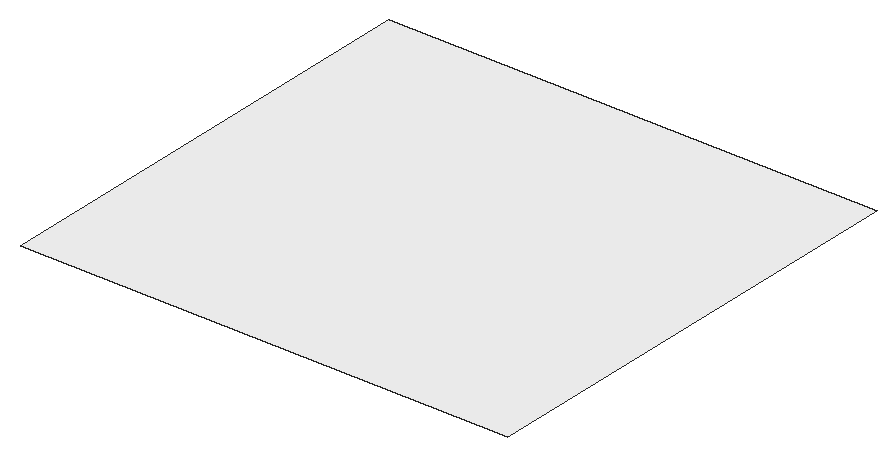
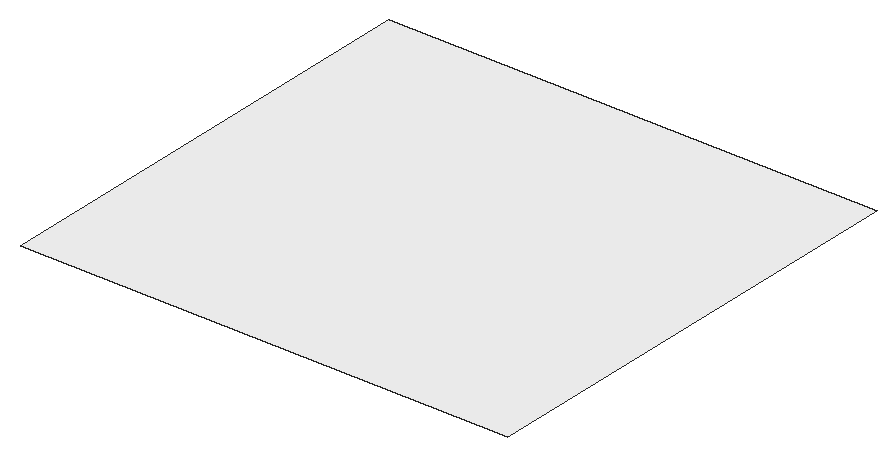
# SketchUp Ruby script. Lengths in inches.
U = 1.inch
M = Sketchup.active_model
def pt(a) = Geom::Point3d.new(a.map { |v| v * U })
def face(e, loops, mat)
  f = e.add_face(loops[0].map { |a| pt(a) })
  loops[1..].each { |l| e.add_face(l.map { |a| pt(a) }).erase! }
  f.material = f.back_material = mat if mat
  f
end
# faces: each face lists its corners as indices into pts; further lists are holes
def faces(e, pts, list, mat = nil) = list.each { |f| face(e, (f[0].is_a?(Array) ? f : [f]).map { |l| l.map { |i| pts[i] } }, mat) }
# xy, xz, yz: faces in a plane at the given z, y or x. An outline is a flat list of corners, or four numbers for a rectangle; further outlines are holes
def ring(l) = l.size == 4 ? [[l[0], l[1]], [l[2], l[1]], [l[2], l[3]], [l[0], l[3]]] : l.each_slice(2).to_a
def flat(e, list, mat, &to3) = list.each { |f| face(e, (f[0].is_a?(Array) ? f : [f]).map { |l| ring(l).map { |u, v| to3.(u, v) } }, mat) }
def xy(e, z, list, mat = nil) = flat(e, list, mat) { |x, y| [x, y, z] }
def xz(e, y, list, mat = nil) = flat(e, list, mat) { |x, z| [x, y, z] }
def yz(e, x, list, mat = nil) = flat(e, list, mat) { |y, z| [x, y, z] }
def lines(e, pts, list) = list.each { |a, b| e.add_line(pt(pts[a]), pt(pts[b])) }
# prism: a flat outline (further loops are holes) pulled along v
def prism(e, loops, v, mat = nil)
  f = face(e, loops, mat); d = Geom::Vector3d.new(v.map { |x| x * U })
  f.pushpull(f.normal.samedirection?(d) ? d.length : -d.length)
end
def box(e, o, s, mat = nil) = prism(e, [[o, [o[0] + s[0], o[1], o[2]], [o[0] + s[0], o[1] + s[1], o[2]], [o[0], o[1] + s[1], o[2]]]], [0, 0, s[2]], mat)
def at(x, y, z, deg = 0) = Geom::Transformation.translation(pt([x, y, z])) * Geom::Transformation.rotation(ORIGIN, Z_AXIS, deg.degrees)
def axes(o, x, y, z) = Geom::Transformation.new([*x, 0, *y, 0, *z, 0, *pt(o).to_a, 1])
def part(name) = M.definitions.add(name)
# library, detail: a bought-in or finely detailed component or shape, given as its bounding box
def library(name, o, s) = part(name).tap { |d| box(d.entities, o, s) }
def detail(e, o, s) = box(e.add_group.entities, o, s)
def put(e, d, t, mat = nil) = e.add_instance(d, t).tap { |i| i.material = mat if mat }
def group(e, t, mat = nil) = e.add_group.tap { |g| g.transformation = t; g.material = mat if mat }.entities
root = M.entities
M.materials.add("Dado").color = [252, 229, 201]
M.materials.add("[Color M00]").color = [255, 255, 255]
xy(root,120,[[29,128,114,133]],"[Color M00]")
xy(root,121,[[29,20,114,20,114,133,112.5,133,112.5,21.5,30.5,21.5,30.5,133,29,133]],"[Color M00]")
xy(root,122,[[14.87,17,14.68,17.02,14.5,17.04,14.3125,17.08,14.13,17.13,13.95,17.1875,13.78,17.26,13.61,17.34,13.44,17.43,13.14,17.65,12.99,17.77,12.86,17.9,12.73,18.04,12.61,18.1875,12.5,18.34,12.4,18.5,12.3125,18.67,12.23,18.84,12.17,19.02,12.11,19.19,12.07,19.38,12.03,19.5625,12.01,19.75,12,19.9375,12,20.13,12.02,20.32,12.04,20.5,12.08,20.6875,12.13,20.87,12.1875,21.05,12.26,21.22,12.34,21.39,12.43,21.56,12.65,21.86,12.77,22.01,12.9,22.14,13.04,22.27,13.1875,22.39,13.34,22.5,13.5,22.6,13.67,22.6875,13.84,22.77,14.02,22.83,14.19,22.89,14.38,22.93,14.5625,22.97,14.75,22.99,14.9375,23,15.13,23,15.32,22.98,15.5,22.96,15.6875,22.92,15.87,22.87,16.05,22.8125,16.22,22.74,16.39,22.66,16.56,22.57,16.86,22.35,17.01,22.23,17.14,22.1,17.27,21.96,17.39,21.8125,17.5,21.66,17.6,21.5,17.6875,21.33,17.77,21.16,17.83,20.98,17.89,20.81,17.93,20.62,17.97,20.4375,17.99,20.25,18,20.0625,18,19.87,17.98,19.68,17.96,19.5,17.92,19.3125,17.87,19.13,17.8125,18.95,17.74,18.78,17.66,18.61,17.57,18.44,17.35,18.14,17.23,17.99,17.1,17.86,16.96,17.73,16.8125,17.61,16.66,17.5,16.5,17.4,16.33,17.3125,16.16,17.23,15.98,17.17,15.81,17.11,15.62,17.07,15.4375,17.03,15.25,17.01,15.0625,17],[127.87,17,127.68,17.02,127.5,17.04,127.3125,17.08,127.13,17.13,126.95,17.1875,126.78,17.26,126.61,17.34,126.44,17.43,126.14,17.65,125.99,17.77,125.86,17.9,125.73,18.04,125.61,18.1875,125.5,18.34,125.4,18.5,125.3125,18.67,125.23,18.84,125.17,19.02,125.11,19.19,125.07,19.38,125.03,19.5625,125.01,19.75,125,19.9375,125,20.13,125.02,20.32,125.04,20.5,125.08,20.6875,125.13,20.87,125.1875,21.05,125.26,21.22,125.34,21.39,125.43,21.56,125.65,21.86,125.77,22.01,125.9,22.14,126.04,22.27,126.1875,22.39,126.34,22.5,126.5,22.6,126.67,22.6875,126.84,22.77,127.02,22.83,127.19,22.89,127.38,22.93,127.5625,22.97,127.75,22.99,127.9375,23,128.13,23,128.32,22.98,128.5,22.96,128.6875,22.92,128.87,22.87,129.05,22.8125,129.22,22.74,129.39,22.66,129.56,22.57,129.86,22.35,130.01,22.23,130.14,22.1,130.27,21.96,130.39,21.8125,130.5,21.66,130.6,21.5,130.6875,21.33,130.77,21.16,130.83,20.98,130.89,20.81,130.93,20.62,130.97,20.4375,130.99,20.25,131,20.0625,131,19.87,130.98,19.68,130.96,19.5,130.92,19.3125,130.87,19.13,130.8125,18.95,130.74,18.78,130.66,18.61,130.57,18.44,130.35,18.14,130.23,17.99,130.1,17.86,129.96,17.73,129.8125,17.61,129.66,17.5,129.5,17.4,129.33,17.3125,129.16,17.23,128.98,17.17,128.81,17.11,128.62,17.07,128.4375,17.03,128.25,17.01,128.0625,17],[14.87,61,14.68,61.02,14.5,61.04,14.3125,61.08,14.13,61.13,13.95,61.1875,13.78,61.26,13.61,61.34,13.44,61.43,13.14,61.65,12.99,61.77,12.86,61.9,12.73,62.04,12.61,62.1875,12.5,62.34,12.4,62.5,12.3125,62.67,12.23,62.84,12.17,63.02,12.11,63.19,12.07,63.38,12.03,63.5625,12.01,63.75,12,63.9375,12,64.13,12.02,64.32,12.04,64.5,12.08,64.6875,12.13,64.87,12.1875,65.05,12.26,65.22,12.34,65.39,12.43,65.56,12.65,65.86,12.77,66.01,12.9,66.14,13.04,66.27,13.1875,66.39,13.34,66.5,13.5,66.6,13.67,66.6875,13.84,66.77,14.02,66.83,14.19,66.89,14.38,66.93,14.5625,66.97,14.75,66.99,14.9375,67,15.13,67,15.32,66.98,15.5,66.96,15.6875,66.92,15.87,66.87,16.05,66.8125,16.22,66.74,16.39,66.66,16.56,66.57,16.86,66.35,17.01,66.23,17.14,66.1,17.27,65.96,17.39,65.8125,17.5,65.66,17.6,65.5,17.6875,65.33,17.77,65.16,17.83,64.98,17.89,64.81,17.93,64.62,17.97,64.4375,17.99,64.25,18,64.0625,18,63.87,17.98,63.68,17.96,63.5,17.92,63.3125,17.87,63.13,17.8125,62.95,17.74,62.78,17.66,62.61,17.57,62.44,17.35,62.14,17.23,61.99,17.1,61.86,16.96,61.73,16.8125,61.61,16.66,61.5,16.5,61.4,16.33,61.3125,16.16,61.23,15.98,61.17,15.81,61.11,15.62,61.07,15.4375,61.03,15.25,61.01,15.0625,61],[127.87,61,127.68,61.02,127.5,61.04,127.3125,61.08,127.13,61.13,126.95,61.1875,126.78,61.26,126.61,61.34,126.44,61.43,126.14,61.65,125.99,61.77,125.86,61.9,125.73,62.04,125.61,62.1875,125.5,62.34,125.4,62.5,125.3125,62.67,125.23,62.84,125.17,63.02,125.11,63.19,125.07,63.38,125.03,63.5625,125.01,63.75,125,63.9375,125,64.13,125.02,64.32,125.04,64.5,125.08,64.6875,125.13,64.87,125.1875,65.05,125.26,65.22,125.34,65.39,125.43,65.56,125.65,65.86,125.77,66.01,125.9,66.14,126.04,66.27,126.1875,66.39,126.34,66.5,126.5,66.6,126.67,66.6875,126.84,66.77,127.02,66.83,127.19,66.89,127.38,66.93,127.5625,66.97,127.75,66.99,127.9375,67,128.13,67,128.32,66.98,128.5,66.96,128.6875,66.92,128.87,66.87,129.05,66.8125,129.22,66.74,129.39,66.66,129.56,66.57,129.86,66.35,130.01,66.23,130.14,66.1,130.27,65.96,130.39,65.8125,130.5,65.66,130.6,65.5,130.6875,65.33,130.77,65.16,130.83,64.98,130.89,64.81,130.93,64.62,130.97,64.4375,130.99,64.25,131,64.0625,131,63.87,130.98,63.68,130.96,63.5,130.92,63.3125,130.87,63.13,130.8125,62.95,130.74,62.78,130.66,62.61,130.57,62.44,130.35,62.14,130.23,61.99,130.1,61.86,129.96,61.73,129.8125,61.61,129.66,61.5,129.5,61.4,129.33,61.3125,129.16,61.23,128.98,61.17,128.81,61.11,128.62,61.07,128.4375,61.03,128.25,61.01,128.0625,61],[14.87,105,14.68,105.02,14.5,105.04,14.3125,105.08,14.13,105.13,13.95,105.1875,13.78,105.26,13.61,105.34,13.44,105.43,13.14,105.65,12.99,105.77,12.86,105.9,12.73,106.04,12.61,106.1875,12.5,106.34,12.4,106.5,12.3125,106.67,12.23,106.84,12.17,107.02,12.11,107.19,12.07,107.38,12.03,107.5625,12.01,107.75,12,107.9375,12,108.13,12.02,108.32,12.04,108.5,12.08,108.6875,12.13,108.87,12.1875,109.05,12.26,109.22,12.34,109.39,12.43,109.56,12.65,109.86,12.77,110.01,12.9,110.14,13.04,110.27,13.1875,110.39,13.34,110.5,13.5,110.6,13.67,110.6875,13.84,110.77,14.02,110.83,14.19,110.89,14.38,110.93,14.5625,110.97,14.75,110.99,14.9375,111,15.13,111,15.32,110.98,15.5,110.96,15.6875,110.92,15.87,110.87,16.05,110.8125,16.22,110.74,16.39,110.66,16.56,110.57,16.86,110.35,17.01,110.23,17.14,110.1,17.27,109.96,17.39,109.8125,17.5,109.66,17.6,109.5,17.6875,109.33,17.77,109.16,17.83,108.98,17.89,108.81,17.93,108.62,17.97,108.4375,17.99,108.25,18,108.0625,18,107.87,17.98,107.68,17.96,107.5,17.92,107.3125,17.87,107.13,17.8125,106.95,17.74,106.78,17.66,106.61,17.57,106.44,17.35,106.14,17.23,105.99,17.1,105.86,16.96,105.73,16.8125,105.61,16.66,105.5,16.5,105.4,16.33,105.3125,16.16,105.23,15.98,105.17,15.81,105.11,15.62,105.07,15.4375,105.03,15.25,105.01,15.0625,105],
  [127.87,105,127.68,105.02,127.5,105.04,127.3125,105.08,127.13,105.13,126.95,105.1875,126.78,105.26,126.61,105.34,126.44,105.43,126.14,105.65,125.99,105.77,125.86,105.9,125.73,106.04,125.61,106.1875,125.5,106.34,125.4,106.5,125.3125,106.67,125.23,106.84,125.17,107.02,125.11,107.19,125.07,107.38,125.03,107.5625,125.01,107.75,125,107.9375,125,108.13,125.02,108.32,125.04,108.5,125.08,108.6875,125.13,108.87,125.1875,109.05,125.26,109.22,125.34,109.39,125.43,109.56,125.65,109.86,125.77,110.01,125.9,110.14,126.04,110.27,126.1875,110.39,126.34,110.5,126.5,110.6,126.67,110.6875,126.84,110.77,127.02,110.83,127.19,110.89,127.38,110.93,127.5625,110.97,127.75,110.99,127.9375,111,128.13,111,128.32,110.98,128.5,110.96,128.6875,110.92,128.87,110.87,129.05,110.8125,129.22,110.74,129.39,110.66,129.56,110.57,129.86,110.35,130.01,110.23,130.14,110.1,130.27,109.96,130.39,109.8125,130.5,109.66,130.6,109.5,130.6875,109.33,130.77,109.16,130.83,108.98,130.89,108.81,130.93,108.62,130.97,108.4375,130.99,108.25,131,108.0625,131,107.87,130.98,107.68,130.96,107.5,130.92,107.3125,130.87,107.13,130.8125,106.95,130.74,106.78,130.66,106.61,130.57,106.44,130.35,106.14,130.23,105.99,130.1,105.86,129.96,105.73,129.8125,105.61,129.66,105.5,129.5,105.4,129.33,105.3125,129.16,105.23,128.98,105.17,128.81,105.11,128.62,105.07,128.4375,105.03,128.25,105.01,128.0625,105]],"[Color M00]")
xy(root,123,[[[21,12,122,141],[30.5,21.5,112.5,133]],[30.5,21.5,112.5,133]],"[Color M00]")
xy(root,126,[[0,0,162,153]],"[Color M00]")
xz(root,17,[[14.87,120,15.0625,122]],"[Color M00]")
xz(root,21.5,[[30.5,121,112.5,123]],"[Color M00]")
xz(root,23,[[14.9375,120,15.13,122]],"[Color M00]")
xz(root,61,[[14.87,120,15.0625,122]],"[Color M00]")
xz(root,67,[[14.9375,120,15.13,122]],"[Color M00]")
xz(root,105,[[14.87,120,15.0625,122]],"[Color M00]")
xz(root,111,[[14.9375,120,15.13,122],[127.9375,120,128.13,122]],"[Color M00]")
yz(root,12,[[19.9375,120,20.13,122],[63.9375,120,64.13,122],[107.9375,120,108.13,122]],"[Color M00]")
yz(root,18,[[19.87,120,20.0625,122],[63.87,120,64.0625,122],[107.87,120,108.0625,122]],"[Color M00]")
yz(root,30.5,[[21.5,121,133,123]],"[Color M00]")
yz(root,112.5,[[21.5,121,133,123]],"[Color M00]")
p = [[14.5,17.04,120],[14.3125,17.08,120],[14.3125,17.08,122],[14.5,17.04,122],[14.68,17.02,120],[14.68,17.02,122],
  [14.87,17,120],[14.87,17,122],[15.25,17.01,120],[15.0625,17,120],[15.0625,17,122],[15.25,17.01,122],
  [15.4375,17.03,120],[15.4375,17.03,122],[15.62,17.07,120],[15.62,17.07,122],[14.13,17.13,120],[13.95,17.1875,120],
  [13.95,17.1875,122],[14.13,17.13,122],[15.81,17.11,120],[15.81,17.11,122],[15.98,17.17,120],[15.98,17.17,122],
  [13.78,17.26,120],[13.78,17.26,122],[16.16,17.23,120],[16.16,17.23,122],[16.33,17.3125,120],[16.33,17.3125,122],
  [13.61,17.34,120],[13.44,17.43,120],[13.44,17.43,122],[13.61,17.34,122],[16.5,17.4,120],[16.5,17.4,122],
  [13.29,17.54,120],[13.29,17.54,122],[16.66,17.5,120],[16.66,17.5,122],[13.14,17.65,120],[13.14,17.65,122],
  [16.8125,17.61,120],[16.8125,17.61,122],[12.99,17.77,120],[12.99,17.77,122],[16.96,17.73,120],[16.96,17.73,122],
  [17.1,17.86,120],[17.1,17.86,122],[12.86,17.9,120],[12.86,17.9,122],[12.73,18.04,120],[12.73,18.04,122],
  [17.23,17.99,120],[17.23,17.99,122],[12.61,18.1875,120],[12.61,18.1875,122],[17.35,18.14,120],[17.35,18.14,122],
  [17.46,18.29,120],[17.46,18.29,122],[12.5,18.34,120],[12.5,18.34,122],[12.4,18.5,120],[12.4,18.5,122],
  [17.57,18.44,120],[17.57,18.44,122],[17.66,18.61,120],[17.66,18.61,122],[12.3125,18.67,120],[12.3125,18.67,122],
  [17.74,18.78,120],[17.74,18.78,122],[12.23,18.84,120],[12.23,18.84,122],[12.17,19.02,120],[12.17,19.02,122],
  [17.8125,18.95,120],[17.8125,18.95,122],[12.11,19.19,120],[12.11,19.19,122],[17.87,19.13,120],[17.87,19.13,122],
  [17.92,19.3125,120],[17.92,19.3125,122],[12.07,19.38,120],[12.07,19.38,122],[17.96,19.5,120],[17.96,19.5,122],
  [12.03,19.5625,120],[12.03,19.5625,122],[17.98,19.68,120],[17.98,19.68,122],[12.01,19.75,120],[12.01,19.75,122],
  [18,19.87,120],[18,19.87,122],[12,19.9375,120],[12,19.9375,122],[12,20.13,120],[12.02,20.32,120],
  [12.02,20.32,122],[12,20.13,122],[17.99,20.25,120],[18,20.0625,120],[18,20.0625,122],[17.99,20.25,122],
  [17.97,20.4375,120],[17.97,20.4375,122],[12.04,20.5,120],[12.04,20.5,122],[17.93,20.62,120],[17.93,20.62,122],
  [12.08,20.6875,120],[12.08,20.6875,122],[17.89,20.81,120],[17.89,20.81,122],[12.13,20.87,120],[12.13,20.87,122],
  [17.83,20.98,120],[17.83,20.98,122],[12.1875,21.05,120],[12.1875,21.05,122],[12.26,21.22,120],[12.26,21.22,122],
  [17.77,21.16,120],[17.77,21.16,122],[12.34,21.39,120],[12.34,21.39,122],[17.6875,21.33,120],[17.6875,21.33,122],
  [17.6,21.5,120],[17.6,21.5,122],[12.43,21.56,120],[12.43,21.56,122],[17.5,21.66,120],[17.5,21.66,122],
  [12.54,21.71,120],[12.54,21.71,122],[12.65,21.86,120],[12.65,21.86,122],[17.39,21.8125,120],[17.39,21.8125,122],
  [17.27,21.96,120],[17.27,21.96,122],[12.77,22.01,120],[12.77,22.01,122],[12.9,22.14,120],[12.9,22.14,122],
  [17.14,22.1,120],[17.14,22.1,122],[13.04,22.27,120],[13.04,22.27,122],[17.01,22.23,120],[17.01,22.23,122],
  [16.86,22.35,120],[16.86,22.35,122],[13.1875,22.39,120],[13.1875,22.39,122],[13.34,22.5,120],[13.34,22.5,122],
  [16.71,22.46,120],[16.71,22.46,122],[13.5,22.6,120],[13.5,22.6,122],[16.56,22.57,120],[16.56,22.57,122],
  [13.67,22.6875,120],[13.67,22.6875,122],[16.39,22.66,120],[16.39,22.66,122],[13.84,22.77,120],[13.84,22.77,122],
  [16.05,22.8125,120],[16.22,22.74,120],[16.22,22.74,122],[16.05,22.8125,122],[14.02,22.83,120],[14.02,22.83,122],
  [14.19,22.89,120],[14.19,22.89,122],[15.87,22.87,120],[15.87,22.87,122],[14.38,22.93,120],[14.38,22.93,122],
  [14.5625,22.97,120],[14.5625,22.97,122],[15.5,22.96,120],[15.6875,22.92,120],[15.6875,22.92,122],[15.5,22.96,122],
  [14.75,22.99,120],[14.75,22.99,122],[14.9375,23,120],[14.9375,23,122],[15.13,23,120],[15.32,22.98,120],
  [15.32,22.98,122],[15.13,23,122],[14.5,61.04,120],[14.3125,61.08,120],[14.3125,61.08,122],[14.5,61.04,122],
  [14.68,61.02,120],[14.68,61.02,122],[14.87,61,120],[14.87,61,122],[15.25,61.01,120],[15.0625,61,120],
  [15.0625,61,122],[15.25,61.01,122],[15.4375,61.03,120],[15.4375,61.03,122],[15.62,61.07,120],[15.62,61.07,122],
  [14.13,61.13,120],[13.95,61.1875,120],[13.95,61.1875,122],[14.13,61.13,122],[15.81,61.11,120],[15.81,61.11,122],
  [15.98,61.17,120],[15.98,61.17,122],[13.78,61.26,120],[13.78,61.26,122],[16.16,61.23,120],[16.16,61.23,122],
  [16.33,61.3125,120],[16.33,61.3125,122],[13.61,61.34,120],[13.44,61.43,120],[13.44,61.43,122],[13.61,61.34,122],
  [16.5,61.4,120],[16.5,61.4,122],[13.29,61.54,120],[13.29,61.54,122],[16.66,61.5,120],[16.66,61.5,122],
  [13.14,61.65,120],[13.14,61.65,122],[16.8125,61.61,120],[16.8125,61.61,122],[12.99,61.77,120],[12.99,61.77,122],
  [16.96,61.73,120],[16.96,61.73,122],[17.1,61.86,120],[17.1,61.86,122],[12.86,61.9,120],[12.86,61.9,122],
  [12.73,62.04,120],[12.73,62.04,122],[17.23,61.99,120],[17.23,61.99,122],[12.61,62.1875,120],[12.61,62.1875,122],
  [17.35,62.14,120],[17.35,62.14,122],[17.46,62.29,120],[17.46,62.29,122],[12.5,62.34,120],[12.5,62.34,122],
  [12.4,62.5,120],[12.4,62.5,122],[17.57,62.44,120],[17.57,62.44,122],[17.66,62.61,120],[17.66,62.61,122],
  [12.3125,62.67,120],[12.3125,62.67,122],[17.74,62.78,120],[17.74,62.78,122],[12.23,62.84,120],[12.23,62.84,122],
  [12.17,63.02,120],[12.17,63.02,122],[17.8125,62.95,120],[17.8125,62.95,122],[12.11,63.19,120],[12.11,63.19,122],
  [17.87,63.13,120],[17.87,63.13,122],[17.92,63.3125,120],[17.92,63.3125,122],[12.07,63.38,120],[12.07,63.38,122],
  [17.96,63.5,120],[17.96,63.5,122],[12.03,63.5625,120],[12.03,63.5625,122],[17.98,63.68,120],[17.98,63.68,122],
  [12.01,63.75,120],[12.01,63.75,122],[18,63.87,120],[18,63.87,122],[12,63.9375,120],[12,63.9375,122],
  [12,64.13,120],[12.02,64.32,120],[12.02,64.32,122],[12,64.13,122],[17.99,64.25,120],[18,64.0625,120],
  [18,64.0625,122],[17.99,64.25,122],[17.97,64.4375,120],[17.97,64.4375,122],[12.04,64.5,120],[12.04,64.5,122],
  [17.93,64.62,120],[17.93,64.62,122],[12.08,64.6875,120],[12.08,64.6875,122],[17.89,64.81,120],[17.89,64.81,122],
  [12.13,64.87,120],[12.13,64.87,122],[17.83,64.98,120],[17.83,64.98,122],[12.1875,65.05,120],[12.1875,65.05,122],
  [12.26,65.22,120],[12.26,65.22,122],[17.77,65.16,120],[17.77,65.16,122],[12.34,65.39,120],[12.34,65.39,122],
  [17.6875,65.33,120],[17.6875,65.33,122],[17.6,65.5,120],[17.6,65.5,122],[12.43,65.56,120],[12.43,65.56,122],
  [17.5,65.66,120],[17.5,65.66,122],[12.54,65.71,120],[12.54,65.71,122],[12.65,65.86,120],[12.65,65.86,122],
  [17.39,65.8125,120],[17.39,65.8125,122],[17.27,65.96,120],[17.27,65.96,122],[12.77,66.01,120],[12.77,66.01,122],
  [12.9,66.14,120],[12.9,66.14,122],[17.14,66.1,120],[17.14,66.1,122],[13.04,66.27,120],[13.04,66.27,122],
  [17.01,66.23,120],[17.01,66.23,122],[16.86,66.35,120],[16.86,66.35,122],[13.1875,66.39,120],[13.1875,66.39,122],
  [13.34,66.5,120],[13.34,66.5,122],[16.71,66.46,120],[16.71,66.46,122],[13.5,66.6,120],[13.5,66.6,122],
  [16.56,66.57,120],[16.56,66.57,122],[13.67,66.6875,120],[13.67,66.6875,122],[16.39,66.66,120],[16.39,66.66,122],
  [13.84,66.77,120],[13.84,66.77,122],[16.05,66.8125,120],[16.22,66.74,120],[16.22,66.74,122],[16.05,66.8125,122],
  [14.02,66.83,120],[14.02,66.83,122],[14.19,66.89,120],[14.19,66.89,122],[15.87,66.87,120],[15.87,66.87,122],
  [14.38,66.93,120],[14.38,66.93,122],[14.5625,66.97,120],[14.5625,66.97,122],[15.5,66.96,120],[15.6875,66.92,120],
  [15.6875,66.92,122],[15.5,66.96,122],[14.75,66.99,120],[14.75,66.99,122],[14.9375,67,120],[14.9375,67,122],
  [15.13,67,120],[15.32,66.98,120],[15.32,66.98,122],[15.13,67,122],[14.5,105.04,120],[14.3125,105.08,120],
  [14.3125,105.08,122],[14.5,105.04,122],[14.68,105.02,120],[14.68,105.02,122],[14.87,105,120],[14.87,105,122],
  [15.25,105.01,120],[15.0625,105,120],[15.0625,105,122],[15.25,105.01,122],[15.4375,105.03,120],[15.4375,105.03,122],
  [15.62,105.07,120],[15.62,105.07,122],[14.13,105.13,120],[13.95,105.1875,120],[13.95,105.1875,122],[14.13,105.13,122],
  [15.81,105.11,120],[15.81,105.11,122],[15.98,105.17,120],[15.98,105.17,122],[13.78,105.26,120],[13.78,105.26,122],
  [16.16,105.23,120],[16.16,105.23,122],[16.33,105.3125,120],[16.33,105.3125,122],[13.61,105.34,120],[13.44,105.43,120],
  [13.44,105.43,122],[13.61,105.34,122],[16.5,105.4,120],[16.5,105.4,122],[13.29,105.54,120],[13.29,105.54,122],
  [16.66,105.5,120],[16.66,105.5,122],[13.14,105.65,120],[13.14,105.65,122],[16.8125,105.61,120],[16.8125,105.61,122],
  [12.99,105.77,120],[12.99,105.77,122],[16.96,105.73,120],[16.96,105.73,122],[17.1,105.86,120],[17.1,105.86,122],
  [12.86,105.9,120],[12.86,105.9,122],[12.73,106.04,120],[12.73,106.04,122],[17.23,105.99,120],[17.23,105.99,122],
  [12.61,106.1875,120],[12.61,106.1875,122],[17.35,106.14,120],[17.35,106.14,122],[17.46,106.29,120],[17.46,106.29,122],
  [12.5,106.34,120],[12.5,106.34,122],[12.4,106.5,120],[12.4,106.5,122],[17.57,106.44,120],[17.57,106.44,122],
  [17.66,106.61,120],[17.66,106.61,122],[12.3125,106.67,120],[12.3125,106.67,122],[17.74,106.78,120],[17.74,106.78,122],
  [12.23,106.84,120],[12.23,106.84,122],[12.17,107.02,120],[12.17,107.02,122],[17.8125,106.95,120],[17.8125,106.95,122],
  [12.11,107.19,120],[12.11,107.19,122],[17.87,107.13,120],[17.87,107.13,122],[17.92,107.3125,120],[17.92,107.3125,122],
  [12.07,107.38,120],[12.07,107.38,122],[17.96,107.5,120],[17.96,107.5,122],[12.03,107.5625,120],[12.03,107.5625,122],
  [17.98,107.68,120],[17.98,107.68,122],[12.01,107.75,120],[12.01,107.75,122],[18,107.87,120],[18,107.87,122],
  [12,107.9375,120],[12,107.9375,122],[12,108.13,120],[12.02,108.32,120],[12.02,108.32,122],[12,108.13,122],
  [17.99,108.25,120],[18,108.0625,120],[18,108.0625,122],[17.99,108.25,122],[17.97,108.4375,120],[17.97,108.4375,122],
  [12.04,108.5,120],[12.04,108.5,122],[17.93,108.62,120],[17.93,108.62,122],[12.08,108.6875,120],[12.08,108.6875,122],
  [17.89,108.81,120],[17.89,108.81,122],[12.13,108.87,120],[12.13,108.87,122],[17.83,108.98,120],[17.83,108.98,122],
  [12.1875,109.05,120],[12.1875,109.05,122],[12.26,109.22,120],[12.26,109.22,122],[17.77,109.16,120],[17.77,109.16,122],
  [12.34,109.39,120],[12.34,109.39,122],[17.6875,109.33,120],[17.6875,109.33,122],[17.6,109.5,120],[17.6,109.5,122],
  [12.43,109.56,120],[12.43,109.56,122],[17.5,109.66,120],[17.5,109.66,122],[12.54,109.71,120],[12.54,109.71,122],
  [12.65,109.86,120],[12.65,109.86,122],[17.39,109.8125,120],[17.39,109.8125,122],[17.27,109.96,120],[17.27,109.96,122],
  [12.77,110.01,120],[12.77,110.01,122],[125.65,109.86,120],[125.77,110.01,120],[125.77,110.01,122],[125.65,109.86,122],
  [12.9,110.14,120],[12.9,110.14,122],[17.14,110.1,120],[17.14,110.1,122],[125.9,110.14,120],[125.9,110.14,122],
  [13.04,110.27,120],[13.04,110.27,122],[17.01,110.23,120],[17.01,110.23,122],[126.04,110.27,120],[126.04,110.27,122],
  [16.86,110.35,120],[16.86,110.35,122],[13.1875,110.39,120],[13.1875,110.39,122],[126.1875,110.39,120],[126.1875,110.39,122],
  [13.34,110.5,120],[13.34,110.5,122],[16.71,110.46,120],[16.71,110.46,122],[126.34,110.5,120],[126.34,110.5,122],
  [129.71,110.46,120],[129.86,110.35,120],[129.86,110.35,122],[129.71,110.46,122],[13.5,110.6,120],[13.5,110.6,122],
  [16.56,110.57,120],[16.56,110.57,122],[126.5,110.6,120],[126.5,110.6,122],[129.56,110.57,120],[129.56,110.57,122],
  [13.67,110.6875,120],[13.67,110.6875,122],[16.39,110.66,120],[16.39,110.66,122],[126.67,110.6875,120],[126.67,110.6875,122],
  [129.39,110.66,120],[129.39,110.66,122],[13.84,110.77,120],[13.84,110.77,122],[16.05,110.8125,120],[16.22,110.74,120],
  [16.22,110.74,122],[16.05,110.8125,122],[126.84,110.77,120],[126.84,110.77,122],[129.05,110.8125,120],[129.22,110.74,120],
  [129.22,110.74,122],[129.05,110.8125,122],[14.02,110.83,120],[14.02,110.83,122],[14.19,110.89,120],[14.19,110.89,122],
  [15.87,110.87,120],[15.87,110.87,122],[127.02,110.83,120],[127.02,110.83,122],[127.19,110.89,120],[127.19,110.89,122],
  [128.87,110.87,120],[128.87,110.87,122],[14.38,110.93,120],[14.38,110.93,122],[14.5625,110.97,120],[14.5625,110.97,122],
  [15.5,110.96,120],[15.6875,110.92,120],[15.6875,110.92,122],[15.5,110.96,122],[127.38,110.93,120],[127.38,110.93,122],
  [127.5625,110.97,120],[127.5625,110.97,122],[128.5,110.96,120],[128.6875,110.92,120],[128.6875,110.92,122],[128.5,110.96,122],
  [14.75,110.99,120],[14.75,110.99,122],[14.9375,111,120],[14.9375,111,122],[15.13,111,120],[15.32,110.98,120],
  [15.32,110.98,122],[15.13,111,122],[127.75,110.99,120],[127.75,110.99,122],[127.9375,111,120],[127.9375,111,122],
  [128.13,111,120],[128.32,110.98,120],[128.32,110.98,122],[128.13,111,122]]
faces(root,p,[[0,1,2,3],[4,0,3,5],[6,4,5,7],[8,9,10,11],[12,8,11,13],[14,12,13,15],[16,17,18,19],[1,16,19,2],
  [20,14,15,21],[22,20,21,23],[17,24,25,18],[26,22,23,27],[28,26,27,29],[30,31,32,33],[24,30,33,25],[34,28,29,35],
  [31,36,37,32],[38,34,35,39],[36,40,41,37],[42,38,39,43],[40,44,45,41],[46,42,43,47],[48,46,47,49],[44,50,51,45],
  [50,52,53,51],[54,48,49,55],[52,56,57,53],[58,54,55,59],[60,58,59,61],[56,62,63,57],[62,64,65,63],[66,60,61,67],
  [68,66,67,69],[64,70,71,65],[72,68,69,73],[70,74,75,71],[74,76,77,75],[78,72,73,79],[76,80,81,77],[82,78,79,83],
  [84,82,83,85],[80,86,87,81],[88,84,85,89],[86,90,91,87],[92,88,89,93],[90,94,95,91],[96,92,93,97],[94,98,99,95],
  [100,101,102,103],[104,105,106,107],[108,104,107,109],[101,110,111,102],[112,108,109,113],[110,114,115,111],[116,112,113,117],[114,118,119,115],
  [120,116,117,121],[118,122,123,119],[122,124,125,123],[126,120,121,127],[124,128,129,125],[130,126,127,131],[132,130,131,133],[128,134,135,129],
  [136,132,133,137],[134,138,139,135],[138,140,141,139],[142,136,137,143],[144,142,143,145],[140,146,147,141],[146,148,149,147],[150,144,145,151],
  [148,152,153,149],[154,150,151,155],[156,154,155,157],[152,158,159,153],[158,160,161,159],[162,156,157,163],[160,164,165,161],[166,162,163,167],
  [164,168,169,165],[170,166,167,171],[168,172,173,169],[174,175,176,177],[175,170,171,176],[172,178,179,173],[178,180,181,179],[182,174,177,183],
  [180,184,185,181],[184,186,187,185],[188,189,190,191],[189,182,183,190],[186,192,193,187],[192,194,195,193],[196,197,198,199],[197,188,191,198],
  [200,201,202,203],[204,200,203,205],[206,204,205,207],[208,209,210,211],[212,208,211,213],[214,212,213,215],[216,217,218,219],[201,216,219,202],
  [220,214,215,221],[222,220,221,223],[217,224,225,218],[226,222,223,227],[228,226,227,229],[230,231,232,233],[224,230,233,225],[234,228,229,235],
  [231,236,237,232],[238,234,235,239],[236,240,241,237],[242,238,239,243],[240,244,245,241],[246,242,243,247],[248,246,247,249],[244,250,251,245],
  [250,252,253,251],[254,248,249,255],[252,256,257,253],[258,254,255,259],[260,258,259,261],[256,262,263,257],[262,264,265,263],[266,260,261,267],
  [268,266,267,269],[264,270,271,265],[272,268,269,273],[270,274,275,271],[274,276,277,275],[278,272,273,279],[276,280,281,277],[282,278,279,283],
  [284,282,283,285],[280,286,287,281],[288,284,285,289],[286,290,291,287],[292,288,289,293],[290,294,295,291],[296,292,293,297],[294,298,299,295],
  [300,301,302,303],[304,305,306,307],[308,304,307,309],[301,310,311,302],[312,308,309,313],[310,314,315,311],[316,312,313,317],[314,318,319,315],
  [320,316,317,321],[318,322,323,319],[322,324,325,323],[326,320,321,327],[324,328,329,325],[330,326,327,331],[332,330,331,333],[328,334,335,329],
  [336,332,333,337],[334,338,339,335],[338,340,341,339],[342,336,337,343],[344,342,343,345],[340,346,347,341],[346,348,349,347],[350,344,345,351],
  [348,352,353,349],[354,350,351,355],[356,354,355,357],[352,358,359,353],[358,360,361,359],[362,356,357,363],[360,364,365,361],[366,362,363,367],
  [364,368,369,365],[370,366,367,371],[368,372,373,369],[374,375,376,377],[375,370,371,376],[372,378,379,373],[378,380,381,379],[382,374,377,383],
  [380,384,385,381],[384,386,387,385],[388,389,390,391],[389,382,383,390],[386,392,393,387],[392,394,395,393],[396,397,398,399],[397,388,391,398],
  [400,401,402,403],[404,400,403,405],[406,404,405,407],[408,409,410,411],[412,408,411,413],[414,412,413,415],[416,417,418,419],[401,416,419,402],
  [420,414,415,421],[422,420,421,423],[417,424,425,418],[426,422,423,427],[428,426,427,429],[430,431,432,433],[424,430,433,425],[434,428,429,435],
  [431,436,437,432],[438,434,435,439],[436,440,441,437],[442,438,439,443],[440,444,445,441],[446,442,443,447],[448,446,447,449],[444,450,451,445],
  [450,452,453,451],[454,448,449,455],[452,456,457,453],[458,454,455,459],[460,458,459,461],[456,462,463,457],[462,464,465,463],[466,460,461,467],
  [468,466,467,469],[464,470,471,465],[472,468,469,473],[470,474,475,471],[474,476,477,475],[478,472,473,479],[476,480,481,477],[482,478,479,483],
  [484,482,483,485],[480,486,487,481],[488,484,485,489],[486,490,491,487],[492,488,489,493],[490,494,495,491],[496,492,493,497],[494,498,499,495],
  [500,501,502,503],[504,505,506,507],[508,504,507,509],[501,510,511,502],[512,508,509,513],[510,514,515,511],[516,512,513,517],[514,518,519,515],
  [520,516,517,521],[518,522,523,519],[522,524,525,523],[526,520,521,527],[524,528,529,525],[530,526,527,531],[532,530,531,533],[528,534,535,529],
  [536,532,533,537],[534,538,539,535],[538,540,541,539],[542,536,537,543],[544,542,543,545],[540,546,547,541],[548,549,550,551],[546,552,553,547],
  [554,544,545,555],[549,556,557,550],[552,558,559,553],[560,554,555,561],[556,562,563,557],[564,560,561,565],[558,566,567,559],[562,568,569,563],
  [566,570,571,567],[572,564,565,573],[568,574,575,569],[576,577,578,579],[570,580,581,571],[582,572,573,583],[574,584,585,575],[586,576,579,587],
  [580,588,589,581],[590,582,583,591],[584,592,593,585],[594,586,587,595],[588,596,597,589],[598,599,600,601],[599,590,591,600],[592,602,603,593],
  [604,605,606,607],[605,594,595,606],[596,608,609,597],[608,610,611,609],[612,598,601,613],[602,614,615,603],[614,616,617,615],[618,604,607,619],
  [610,620,621,611],[620,622,623,621],[624,625,626,627],[625,612,613,626],[616,628,629,617],[628,630,631,629],[632,633,634,635],[633,618,619,634],
  [622,636,637,623],[636,638,639,637],[640,641,642,643],[641,624,627,642],[630,644,645,631],[644,646,647,645],[648,649,650,651],[649,632,635,650]],"[Color M00]")
g1 = group(root,at(29.58,20.58,121),"Dado")
prism(g1,[[[0,0,0],[0,111.84,0],[0.34,111.84,0],[0.34,0.34,0],[83.5,0.34,0],[83.5,111.84,0],[83.84,111.84,0],[83.84,0,0]]],[0,0,0.3125])
